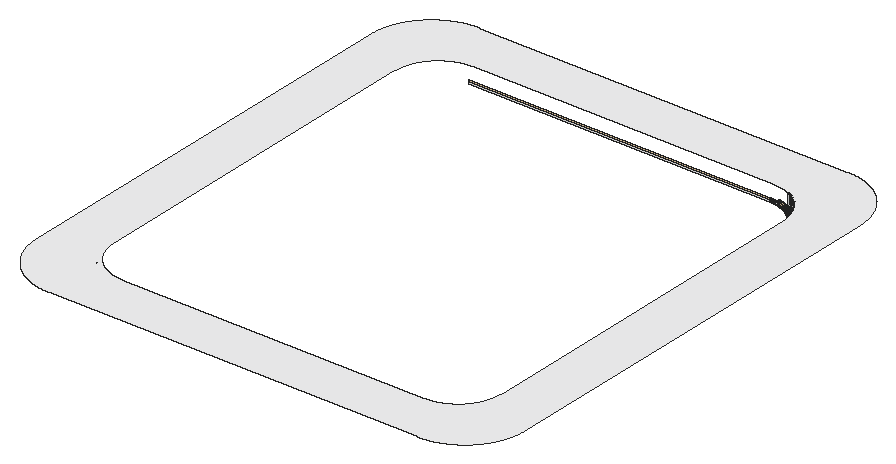
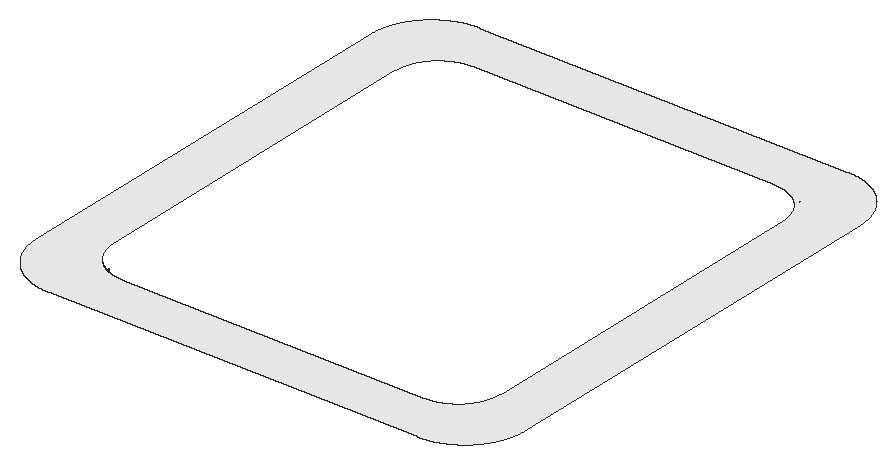
# SketchUp Ruby script. Lengths in inches.
U = 1.inch
M = Sketchup.active_model
def pt(a) = Geom::Point3d.new(a.map { |v| v * U })
def face(e, loops, mat)
  f = e.add_face(loops[0].map { |a| pt(a) })
  loops[1..].each { |l| e.add_face(l.map { |a| pt(a) }).erase! }
  f.material = f.back_material = mat if mat
  f
end
# faces: each face lists its corners as indices into pts; further lists are holes
def faces(e, pts, list, mat = nil) = list.each { |f| face(e, (f[0].is_a?(Array) ? f : [f]).map { |l| l.map { |i| pts[i] } }, mat) }
# xy, xz, yz: faces in a plane at the given z, y or x. An outline is a flat list of corners, or four numbers for a rectangle; further outlines are holes
def ring(l) = l.size == 4 ? [[l[0], l[1]], [l[2], l[1]], [l[2], l[3]], [l[0], l[3]]] : l.each_slice(2).to_a
def flat(e, list, mat, &to3) = list.each { |f| face(e, (f[0].is_a?(Array) ? f : [f]).map { |l| ring(l).map { |u, v| to3.(u, v) } }, mat) }
def xy(e, z, list, mat = nil) = flat(e, list, mat) { |x, y| [x, y, z] }
def xz(e, y, list, mat = nil) = flat(e, list, mat) { |x, z| [x, y, z] }
def yz(e, x, list, mat = nil) = flat(e, list, mat) { |y, z| [x, y, z] }
def lines(e, pts, list) = list.each { |a, b| e.add_line(pt(pts[a]), pt(pts[b])) }
# prism: a flat outline (further loops are holes) pulled along v
def prism(e, loops, v, mat = nil)
  f = face(e, loops, mat); d = Geom::Vector3d.new(v.map { |x| x * U })
  f.pushpull(f.normal.samedirection?(d) ? d.length : -d.length)
end
def box(e, o, s, mat = nil) = prism(e, [[o, [o[0] + s[0], o[1], o[2]], [o[0] + s[0], o[1] + s[1], o[2]], [o[0], o[1] + s[1], o[2]]]], [0, 0, s[2]], mat)
def at(x, y, z, deg = 0) = Geom::Transformation.translation(pt([x, y, z])) * Geom::Transformation.rotation(ORIGIN, Z_AXIS, deg.degrees)
def axes(o, x, y, z) = Geom::Transformation.new([*x, 0, *y, 0, *z, 0, *pt(o).to_a, 1])
def part(name) = M.definitions.add(name)
# library, detail: a bought-in or finely detailed component or shape, given as its bounding box
def library(name, o, s) = part(name).tap { |d| box(d.entities, o, s) }
def detail(e, o, s) = box(e.add_group.entities, o, s)
def put(e, d, t, mat = nil) = e.add_instance(d, t).tap { |i| i.material = mat if mat }
def group(e, t, mat = nil) = e.add_group.tap { |g| g.transformation = t; g.material = mat if mat }.entities
root = M.entities
M.materials.add("False Ceiling Light").color = [254, 223, 179]
M.materials.add("[Quartz Light Grey]").color = [251, 251, 252]
xy(root,120,[[[45.007,44.5,176.993,44.5,177.225,44.501,177.45,44.505,177.675,44.511,177.9,44.519,178.125,44.529,178.35,44.542,178.575,44.558,178.799,44.575,179.023,44.595,179.247,44.618,179.471,44.643,179.695,44.67,179.918,44.699,180.141,44.731,180.363,44.765,180.586,44.801,180.807,44.84,181.029,44.881,181.25,44.924,181.47,44.97,181.69,45.018,181.91,45.068,182.128,45.121,182.347,45.175,182.565,45.233,182.782,45.292,182.998,45.354,183.214,45.418,183.429,45.484,183.644,45.552,183.858,45.623,184.071,45.696,184.283,45.771,184.494,45.848,184.705,45.928,184.915,46.01,185.124,46.094,185.332,46.18,185.539,46.268,185.745,46.359,185.95,46.451,186.154,46.546,186.357,46.643,186.56,46.742,186.761,46.843,186.961,46.947,187.16,47.052,187.358,47.159,187.554,47.269,187.75,47.38,187.944,47.494,188.138,47.61,188.33,47.727,188.52,47.847,188.71,47.969,188.898,48.092,189.085,48.218,189.27,48.345,189.455,48.475,189.637,48.606,189.819,48.739,189.999,48.875,190.177,49.012,190.355,49.151,190.53,49.291,190.705,49.434,190.877,49.578,191.049,49.725,191.218,49.873,191.386,50.022,191.553,50.174,191.718,50.327,191.881,50.482,192.043,50.639,192.203,50.797,192.361,50.957,192.518,51.119,192.673,51.282,192.826,51.447,192.978,51.614,193.127,51.782,193.275,51.951,193.422,52.123,193.566,52.295,193.709,52.47,193.849,52.645,193.988,52.823,194.125,53.001,194.261,53.181,194.394,53.363,194.525,53.545,194.655,53.73,194.782,53.915,194.908,54.102,195.031,54.29,195.153,54.48,195.273,54.67,195.39,54.862,195.506,55.056,195.62,55.25,195.731,55.446,195.841,55.642,195.948,55.84,196.053,56.039,196.157,56.239,196.258,56.44,196.357,56.643,196.454,56.846,196.549,57.05,196.641,57.255,196.732,57.461,196.82,57.668,196.906,57.876,196.99,58.085,197.072,58.295,197.152,58.506,197.229,58.717,197.304,58.929,197.377,59.142,197.448,59.356,197.516,59.571,197.582,59.786,197.646,60.002,197.708,60.218,197.767,60.435,197.825,60.653,197.879,60.872,197.932,61.09,197.982,61.31,198.03,61.53,198.076,61.75,198.119,61.971,198.16,62.193,198.199,62.414,198.235,62.637,198.269,62.859,198.301,63.082,198.33,63.305,198.357,63.529,198.382,63.753,198.405,63.977,198.425,64.201,198.442,64.425,198.458,64.65,198.471,64.875,198.481,65.1,198.489,65.325,198.495,65.55,198.499,65.775,198.5,66.007,198.5,215.993,198.499,216.225,198.495,216.45,198.489,216.675,198.481,216.9,198.471,217.125,198.458,217.35,198.442,217.575,198.425,217.799,198.405,218.023,198.382,218.247,198.357,218.471,198.33,218.695,198.301,218.918,198.269,219.141,198.235,219.363,198.199,219.586,198.16,219.807,198.119,220.029,198.076,220.25,198.03,220.47,197.982,220.69,197.932,220.91,197.879,221.128,197.825,221.347,197.767,221.565,197.708,221.782,197.646,221.998,197.582,222.214,197.516,222.429,197.448,222.644,197.377,222.858,197.304,223.071,197.229,223.283,197.152,223.494,197.072,223.705,196.99,223.915,196.906,224.124,196.82,224.332,196.732,224.539,196.641,224.745,196.549,224.95,196.454,225.154,196.357,225.357,196.258,225.56,196.157,225.761,196.053,225.961,195.948,226.16,195.841,226.358,195.731,226.554,195.62,226.75,195.506,226.944,195.39,227.138,195.273,227.33,195.153,227.52,195.031,227.71,194.908,227.898,194.782,228.085,194.655,228.27,194.525,228.455,194.394,228.637,194.261,228.819,194.125,228.999,193.988,229.177,193.849,229.355,193.709,229.53,193.566,229.705,193.422,229.877,193.275,230.049,193.127,230.218,192.978,230.386,192.826,230.553,192.673,230.718,192.518,230.881,192.361,231.043,192.203,231.203,192.043,231.361,191.881,231.518,191.718,231.673,191.553,231.826,191.386,231.978,191.218,232.127,191.049,232.275,190.877,232.422,190.705,232.566,190.53,232.709,190.355,232.849,190.177,232.988,189.999,233.125,189.819,233.261,189.637,233.394,189.455,233.525,189.27,233.655,189.085,233.782,188.898,233.908,188.71,234.031,188.52,234.153,188.33,234.273,188.138,234.39,187.944,234.506,187.75,234.62,187.554,234.731,187.358,234.841,187.16,234.948,186.961,235.053,186.761,235.157,186.56,235.258,186.357,235.357,186.154,235.454,185.95,235.549,185.745,235.641,185.539,235.732,185.332,235.82,185.124,235.906,184.915,235.99,184.705,236.072,184.494,236.152,184.283,236.229,184.071,236.304,183.858,236.377,183.644,236.448,183.429,236.516,183.214,236.582,182.998,236.646,182.782,236.708,182.565,236.767,182.347,236.825,182.128,236.879,181.91,236.932,181.69,236.982,181.47,237.03,181.25,237.076,181.029,237.119,180.807,237.16,180.586,237.199,180.363,237.235,180.141,237.269,179.918,237.301,179.695,237.33,179.471,237.357,179.247,237.382,179.023,237.405,178.799,237.425,178.575,237.442,178.35,237.458,178.125,237.471,177.9,237.481,177.675,237.489,177.45,237.495,177.225,237.499,176.993,237.5,45.007,237.5,44.775,237.499,44.55,237.495,44.325,237.489,44.1,237.481,43.875,237.471,43.65,237.458,43.425,237.442,43.201,237.425,42.977,237.405,42.753,237.382,42.529,237.357,42.305,237.33,42.082,237.301,41.859,237.269,41.637,237.235,41.414,237.199,41.193,237.16,40.971,237.119,40.75,237.076,40.53,237.03,40.31,236.982,40.09,236.932,39.872,236.879,39.653,236.825,39.435,236.767,39.218,236.708,39.002,236.646,38.786,236.582,38.571,236.516,38.356,236.448,38.142,236.377,37.929,236.304,37.717,236.229,37.506,236.152,37.295,236.072,37.085,235.99,36.876,235.906,36.668,235.82,36.461,235.732,36.255,235.641,36.05,235.549,35.846,235.454,35.643,235.357,35.44,235.258,35.239,235.157,35.039,235.053,34.84,234.948,34.642,234.841,34.446,234.731,34.25,234.62,34.056,234.506,33.862,234.39,33.67,234.273,33.48,234.153,33.29,234.031,33.102,233.908,32.915,233.782,32.73,233.655,32.545,233.525,32.363,233.394,32.181,233.261,32.001,233.125,31.823,232.988,31.645,232.849,31.47,232.709,31.295,232.566,31.123,232.422,30.951,232.275,30.782,232.127,30.614,231.978,30.447,231.826,30.282,231.673,30.119,231.518,29.957,231.361,29.797,231.203,29.639,231.043,29.482,230.881,29.327,230.718,29.174,230.553,29.022,230.386,28.873,230.218,28.725,230.049,28.578,229.877,28.434,229.705,28.291,229.53,28.151,229.355,28.012,229.177,27.875,228.999,27.739,228.819,27.606,228.637,27.475,228.455,27.345,228.27,27.218,228.085,27.092,227.898,26.969,227.71,26.847,227.52,26.727,227.33,26.61,227.138,26.494,226.944,26.38,226.75,26.269,226.554,26.159,226.358,26.052,226.16,25.947,225.961,25.843,225.761,25.742,225.56,25.643,225.357,25.546,225.154,25.451,224.95,25.359,224.745,25.268,224.539,25.18,224.332,25.094,224.124,25.01,223.915,24.928,223.705,24.848,223.494,24.771,223.283,24.696,223.071,24.623,222.858,24.552,222.644,24.484,222.429,24.418,222.214,24.354,221.998,24.292,221.782,24.233,221.565,24.175,221.347,24.121,221.128,24.068,220.91,24.018,220.69,23.97,220.47,23.924,220.25,23.881,220.029,23.84,219.807,23.801,219.586,23.765,219.363,23.731,219.141,23.699,218.918,23.67,218.695,23.643,218.471,23.618,218.247,23.595,218.023,23.575,217.799,23.558,217.575,23.542,217.35,23.529,217.125,23.519,216.9,23.511,216.675,23.505,216.45,23.501,216.225,23.5,215.993,23.5,66.007,23.501,65.775,23.505,65.55,23.511,65.325,23.519,65.1,23.529,64.875,23.542,64.65,23.558,64.425,23.575,64.201,23.595,63.977,23.618,63.753,23.643,63.529,23.67,63.305,23.699,63.082,23.731,62.859,23.765,62.637,23.801,62.414,23.84,62.193,23.881,61.971,23.924,61.75,23.97,61.53,24.018,61.31,24.068,61.09,24.121,60.872,24.175,60.653,24.233,60.435,24.292,60.218,24.354,60.002,24.418,59.786,24.484,59.571,24.552,59.356,24.623,59.142,24.696,58.929,24.771,58.717,24.848,58.506,24.928,58.295,25.01,58.085,25.094,57.876,25.18,57.668,25.268,57.461,25.359,57.255,25.451,57.05,25.546,56.846,25.643,56.643,25.742,56.44,25.843,56.239,25.947,56.039,26.052,55.84,26.159,55.642,26.269,55.446,26.38,55.25,26.494,55.056,26.61,54.862,26.727,54.67,26.847,54.48,26.969,54.29,27.092,54.102,27.218,53.915,27.345,53.73,27.475,53.545,27.606,53.363,27.739,53.181,27.875,53.001,28.012,52.823,28.151,52.645,28.291,52.47,28.434,52.295,28.578,52.123,28.725,51.951,28.873,51.782,29.022,51.614,29.174,51.447,29.327,51.282,29.482,51.119,29.639,50.957,29.797,50.797,29.957,50.639,30.119,50.482,30.282,50.327,30.447,50.174,30.614,50.022,30.782,49.873,30.951,49.725,31.123,49.578,31.295,49.434,31.47,49.291,31.645,49.151,31.823,49.012,32.001,48.875,32.181,48.739,32.363,48.606,32.545,48.475,32.73,48.345,32.915,48.218,33.102,48.092,33.29,47.969,33.48,47.847,33.67,47.727,33.862,47.61,34.056,47.494,34.25,47.38,34.446,47.269,34.642,47.159,34.84,47.052,35.039,46.947,35.239,46.843,35.44,46.742,35.643,46.643,35.846,46.546,36.05,46.451,36.255,46.359,36.461,46.268,36.668,46.18,36.876,46.094,37.085,46.01,37.295,45.928,37.506,45.848,37.717,45.771,37.929,45.696,38.142,45.623,38.356,45.552,38.571,45.484,38.786,45.418,39.002,45.354,39.218,45.292,39.435,45.233,39.653,45.175,39.872,45.121,40.09,45.068,40.31,45.018,40.53,44.97,40.75,44.924,40.971,44.881,41.193,44.84,41.414,44.801,41.637,44.765,41.859,44.731,42.082,44.699,42.305,44.67,42.529,44.643,42.753,44.618,42.977,44.595,43.201,44.575,43.425,44.558,43.65,44.542,43.875,44.529,44.1,44.519,44.325,44.511,44.55,44.505,44.775,44.501],[56.989,62.5,56.796,62.501,56.593,62.505,56.389,62.512,56.186,62.521,55.983,62.533,55.78,62.548,55.577,62.565,55.374,62.585,55.172,62.608,54.97,62.633,54.768,62.661,54.567,62.692,54.366,62.725,54.166,62.761,53.966,62.8,53.767,62.841,53.568,62.885,53.37,62.931,53.172,62.98,52.975,63.032,52.779,63.086,52.583,63.142,52.389,63.202,52.195,63.264,52.002,63.328,51.809,63.395,51.618,63.464,51.428,63.536,51.238,63.611,51.05,63.6875,50.862,63.767,50.676,63.849,50.49,63.933,50.306,64.02,50.123,64.109,49.941,64.2,49.761,64.294,49.581,64.391,49.403,64.489,49.227,64.59,49.051,64.693,48.877,64.799,48.704,64.907,48.533,65.017,48.363,65.129,48.195,65.244,48.028,65.36,47.863,65.479,47.699,65.6,47.537,65.724,47.377,65.849,47.218,65.976,47.061,66.106,46.906,66.237,46.752,66.371,46.6,66.507,46.45,66.644,46.302,66.784,46.156,66.925,46.011,67.068,45.868,67.214,45.728,67.361,45.589,67.51,45.452,67.661,45.317,67.813,45.185,67.967,45.054,68.123,44.925,68.281,44.799,68.441,44.674,68.602,44.552,68.764,44.432,68.929,44.314,69.095,44.198,69.262,44.084,69.431,43.973,69.601,43.863,69.773,43.756,69.946,43.652,70.121,43.549,70.297,43.449,70.474,43.352,70.653,43.257,70.833,43.164,71.014,43.073,71.196,42.985,71.38,42.899,71.564,42.816,71.75,42.735,71.937,42.657,72.125,42.581,72.313,42.507,72.503,42.436,72.694,42.368,72.886,42.302,73.078,42.239,73.272,42.178,73.466,42.119,73.661,42.064,73.857,42.011,74.054,41.96,74.251,41.912,74.449,41.867,74.647,41.824,74.846,41.784,75.046,41.746,75.246,41.712,75.446,41.679,75.647,41.65,75.849,41.623,76.051,41.599,76.253,41.577,76.455,41.558,76.658,41.542,76.861,41.528,77.064,41.517,77.267,41.509,77.47,41.503,77.674,41.5,77.878,41.5,204.011,41.501,204.203,41.505,204.406,41.512,204.609,41.521,204.811,41.533,205.014,41.548,205.216,41.565,205.418,41.585,205.62,41.607,205.822,41.633,206.023,41.66,206.224,41.691,206.425,41.724,206.625,41.759,206.825,41.798,207.024,41.839,207.223,41.882,207.421,41.928,207.618,41.977,207.815,42.028,208.012,42.082,208.207,42.138,208.402,42.197,208.596,42.259,208.79,42.323,208.982,42.389,209.174,42.458,209.365,42.529,209.555,42.603,209.744,42.68,209.932,42.759,210.119,42.84,210.304,42.924,210.489,43.01,210.673,43.098,210.856,43.189,211.037,43.283,211.217,43.378,211.396,43.476,211.574,43.577,211.75,43.679,211.925,43.784,212.099,43.891,212.271,44.001,212.442,44.112,212.611,44.226,212.779,44.342,212.946,44.46,213.111,44.581,213.274,44.703,213.436,44.828,213.596,44.954,213.755,45.083,213.911,45.214,214.066,45.346,214.22,45.481,214.372,45.618,214.521,45.757,214.67,45.897,214.816,46.04,214.96,46.184,215.103,46.33,215.243,46.479,215.382,46.628,215.519,46.78,215.654,46.934,215.786,47.089,215.917,47.245,216.046,47.404,216.172,47.564,216.297,47.726,216.419,47.889,216.54,48.054,216.658,48.221,216.774,48.389,216.888,48.558,216.999,48.729,217.109,48.901,217.216,49.075,217.321,49.25,217.423,49.426,217.524,49.604,217.622,49.783,217.717,49.963,217.811,50.144,217.902,50.327,217.99,50.511,218.076,50.696,218.16,50.881,218.241,51.068,218.32,51.256,218.397,51.445,218.471,51.635,218.542,51.826,218.611,52.018,218.677,52.21,218.741,52.404,218.803,52.598,218.862,52.793,218.918,52.988,218.972,53.185,219.023,53.382,219.072,53.579,219.118,53.777,219.161,53.976,219.202,54.175,219.241,54.375,219.276,54.575,219.309,54.776,219.34,54.977,219.367,55.178,219.393,55.38,219.415,55.582,219.435,55.784,219.452,55.986,219.467,56.189,219.479,56.391,219.488,56.594,219.495,56.797,219.499,56.989,219.5,165.011,219.5,165.203,219.499,165.406,219.495,165.609,219.488,165.811,219.479,166.014,219.467,166.216,219.452,166.418,219.435,166.62,219.415,166.822,219.393,167.023,219.367,167.224,219.34,167.425,219.309,167.625,219.276,167.825,219.241,168.024,219.202,168.223,219.161,168.421,219.118,168.618,219.072,168.815,219.023,169.012,218.972,169.207,218.918,169.402,218.862,169.596,218.803,169.79,218.741,169.982,218.677,170.174,218.611,170.365,218.542,170.555,218.471,170.744,218.397,170.932,218.32,171.119,218.241,171.304,218.16,171.489,218.076,171.673,217.99,171.856,217.902,172.037,217.811,172.217,217.717,172.396,217.622,172.574,217.524,172.75,217.423,172.925,217.321,173.099,217.216,173.271,217.109,173.442,216.999,173.611,216.888,173.779,216.774,173.946,216.658,174.111,216.54,174.274,216.419,174.436,216.297,174.596,216.172,174.755,216.046,174.911,215.917,175.066,215.786,175.22,215.654,175.372,215.519,175.521,215.382,175.67,215.243,175.816,215.103,175.96,214.96,176.103,214.816,176.243,214.67,176.382,214.521,176.519,214.372,176.654,214.22,176.786,214.066,176.917,213.911,177.046,213.755,177.172,213.596,177.297,213.436,177.419,213.274,177.54,213.111,177.658,212.946,177.774,212.779,177.888,212.611,177.999,212.442,178.109,212.271,178.216,212.099,178.321,211.925,178.423,211.75,178.524,211.574,178.622,211.396,178.717,211.217,178.811,211.037,178.902,210.856,178.99,210.673,179.076,210.489,179.16,210.304,179.241,210.119,179.32,209.932,179.397,209.744,179.471,209.555,179.542,209.365,179.611,209.174,179.677,208.982,179.741,208.79,179.803,208.596,179.862,208.402,179.918,208.207,179.972,208.012,180.023,207.815,180.072,207.618,180.118,207.421,180.161,207.223,180.202,207.024,180.241,206.825,180.276,206.625,180.309,206.425,180.34,206.224,180.367,206.023,180.393,205.822,180.415,205.62,180.435,205.418,180.452,205.216,180.467,205.014,180.479,204.811,180.488,204.609,180.495,204.406,180.499,204.203,180.5,204.011,180.5,77.989,180.499,77.797,180.495,77.594,180.488,77.391,180.479,77.189,180.467,76.986,180.452,76.784,180.435,76.582,180.415,76.38,180.393,76.178,180.367,75.977,180.34,75.776,180.309,75.575,180.276,75.375,180.241,75.175,180.202,74.976,180.161,74.777,180.118,74.579,180.072,74.382,180.023,74.185,179.972,73.988,179.918,73.793,179.862,73.598,179.803,73.404,179.741,73.21,179.677,73.018,179.611,72.826,179.542,72.635,179.471,72.445,179.397,72.256,179.32,72.068,179.241,71.881,179.16,71.696,179.076,71.511,178.99,71.327,178.902,71.144,178.811,70.963,178.717,70.783,178.622,70.604,178.524,70.426,178.423,70.25,178.321,70.075,178.216,69.901,178.109,69.729,177.999,69.558,177.888,69.389,177.774,69.221,177.658,69.054,177.54,68.889,177.419,68.726,177.297,68.564,177.172,68.404,177.046,68.245,176.917,68.089,176.786,67.934,176.654,67.78,176.519,67.628,176.382,67.479,176.243,67.33,176.103,67.184,175.96,67.04,175.816,66.897,175.67,66.757,175.521,66.618,175.372,66.481,175.22,66.346,175.066,66.214,174.911,66.083,174.755,65.954,174.596,65.828,174.436,65.703,174.274,65.581,174.111,65.46,173.946,65.342,173.779,65.226,173.611,65.112,173.442,65.001,173.271,64.891,173.099,64.784,172.925,64.679,172.75,64.577,172.574,64.476,172.396,64.378,172.217,64.283,172.037,64.189,171.856,64.098,171.673,64.01,171.489,63.924,171.304,63.84,171.119,63.759,170.932,63.68,170.744,63.603,170.555,63.529,170.365,63.458,170.174,63.389,169.982,63.323,169.79,63.259,169.596,63.197,169.402,63.138,169.207,63.082,169.012,63.028,168.815,62.977,168.618,62.928,168.421,62.882,168.223,62.839,168.024,62.798,167.825,62.759,167.625,62.724,167.425,62.691,167.224,62.66,167.023,62.633,166.822,62.607,166.62,62.585,166.418,62.565,166.216,62.548,166.014,62.533,165.811,62.521,165.609,62.512,165.406,62.505,165.203,62.501,165.011,62.5],[45,66,45,66.063,45.004,66]]],"[Quartz Light Grey]")
xz(root,217.5,[[56.995,115.32,165.005,116.49]],"False Ceiling Light")
xz(root,217.5,[[56.995,115.32,165.005,115.905]],"[Quartz Light Grey]")
p = [[176.025,211.791,115.32],[176.126,211.647,115.32],[176.126,211.647,116.49],[176.025,211.791,116.49],[176.126,211.647,115.32],[176.025,211.791,115.32],
  [176.025,211.791,115.905],[176.126,211.647,115.905],[175.922,211.935,115.32],[175.922,211.935,116.49],[175.922,211.935,115.32],[175.922,211.935,115.905],
  [175.817,212.077,115.32],[175.817,212.077,116.49],[175.817,212.077,115.32],[175.817,212.077,115.905],[175.71,212.218,115.32],[175.71,212.218,116.49],
  [175.71,212.218,115.32],[175.71,212.218,115.905],[175.602,212.358,115.32],[175.602,212.358,116.49],[175.602,212.358,115.32],[175.602,212.358,115.905],
  [175.491,212.496,115.32],[175.491,212.496,116.49],[175.491,212.496,115.32],[175.491,212.496,115.905],[175.379,212.632,115.32],[175.379,212.632,116.49],
  [175.379,212.632,115.32],[175.379,212.632,115.905],[175.266,212.768,115.32],[175.266,212.768,116.49],[175.266,212.768,115.32],[175.266,212.768,115.905],
  [175.15,212.901,115.32],[175.15,212.901,116.49],[175.15,212.901,115.32],[175.15,212.901,115.905],[175.032,213.033,115.32],[175.032,213.033,116.49],
  [175.032,213.033,115.32],[175.032,213.033,115.905],[174.913,213.164,115.32],[174.913,213.164,116.49],[174.913,213.164,115.32],[174.913,213.164,115.905],
  [174.793,213.293,115.32],[174.793,213.293,116.49],[174.793,213.293,115.32],[174.793,213.293,115.905],[174.67,213.42,115.32],[174.67,213.42,116.49],
  [174.67,213.42,115.32],[174.67,213.42,115.905],[176.148,213.272,115.32],[176.026,213.417,115.32],[176.026,213.417,116.49],[176.148,213.272,116.49],
  [174.546,213.546,115.32],[174.546,213.546,116.49],[174.546,213.546,115.32],[174.546,213.546,115.905],[175.902,213.561,115.32],[175.902,213.561,116.49],
  [174.42,213.67,115.32],[174.42,213.67,116.49],[174.42,213.67,115.32],[174.42,213.67,115.905],[175.776,213.702,115.32],[175.776,213.702,116.49],
  [174.293,213.793,115.32],[174.293,213.793,116.49],[174.293,213.793,115.32],[174.293,213.793,115.905],[175.648,213.843,115.32],[175.648,213.843,116.49],
  [174.164,213.913,115.32],[174.164,213.913,116.49],[174.164,213.913,115.32],[174.164,213.913,115.905],[175.518,213.981,115.32],[175.518,213.981,116.49],
  [174.033,214.032,115.32],[174.033,214.032,116.49],[174.033,214.032,115.32],[174.033,214.032,115.905],[173.901,214.15,115.32],[173.901,214.15,116.49],
  [173.901,214.15,115.32],[173.901,214.15,115.905],[175.386,214.118,115.32],[175.386,214.118,116.49],[173.768,214.266,115.32],[173.768,214.266,116.49],
  [173.768,214.266,115.32],[173.768,214.266,115.905],[175.253,214.253,115.32],[175.253,214.253,116.49],[173.632,214.379,115.32],[173.632,214.379,116.49],
  [173.632,214.379,115.32],[173.632,214.379,115.905],[175.118,214.386,115.32],[175.118,214.386,116.49],[173.496,214.491,115.32],[173.496,214.491,116.49],
  [173.496,214.491,115.32],[173.496,214.491,115.905],[174.981,214.518,115.32],[174.981,214.518,116.49],[173.358,214.602,115.32],[173.358,214.602,116.49],
  [173.358,214.602,115.32],[173.358,214.602,115.905],[174.843,214.648,115.32],[174.843,214.648,116.49],[173.218,214.71,115.32],[173.218,214.71,116.49],
  [173.218,214.71,115.32],[173.218,214.71,115.905],[174.702,214.776,115.32],[174.702,214.776,116.49],[173.077,214.817,115.32],[173.077,214.817,116.49],
  [173.077,214.817,115.32],[173.077,214.817,115.905],[176.103,214.816,115.32],[176.243,214.67,115.32],[176.243,214.67,120],[176.103,214.816,120],
  [172.935,214.922,115.32],[172.935,214.922,116.49],[172.935,214.922,115.32],[172.935,214.922,115.905],[174.561,214.902,115.32],[174.561,214.902,116.49],
  [175.96,214.96,115.32],[175.96,214.96,120],[172.791,215.025,115.32],[172.791,215.025,116.49],[172.791,215.025,115.32],[172.791,215.025,115.905],
  [174.417,215.026,115.32],[174.417,215.026,116.49],[172.647,215.126,115.32],[172.647,215.126,116.49],[172.647,215.126,115.32],[172.647,215.126,115.905],
  [174.272,215.148,115.32],[174.272,215.148,116.49],[175.816,215.103,115.32],[175.816,215.103,120],[172.5,215.225,115.32],[172.5,215.225,116.49],
  [172.5,215.225,115.32],[172.5,215.225,115.905],[174.125,215.269,115.32],[174.125,215.269,116.49],[175.67,215.243,115.32],[175.67,215.243,120],
  [172.353,215.322,115.32],[172.353,215.322,116.49],[172.353,215.322,115.32],[172.353,215.322,115.905],[175.521,215.382,115.32],[175.521,215.382,120],
  [172.204,215.417,115.32],[172.204,215.417,116.49],[172.204,215.417,115.32],[172.204,215.417,115.905],[173.977,215.387,115.32],[173.977,215.387,116.49],
  [172.054,215.511,115.32],[172.054,215.511,116.49],[172.054,215.511,115.32],[172.054,215.511,115.905],[173.827,215.504,115.32],[173.827,215.504,116.49],
  [175.372,215.519,115.32],[175.372,215.519,120],[171.902,215.602,115.32],[171.902,215.602,116.49],[171.902,215.602,115.32],[171.902,215.602,115.905],
  [173.676,215.618,115.32],[173.676,215.618,116.49],[175.22,215.654,115.32],[175.22,215.654,120],[171.75,215.691,115.32],[171.75,215.691,116.49],
  [171.75,215.691,115.32],[171.75,215.691,115.905],[173.523,215.731,115.32],[173.523,215.731,116.49],[171.596,215.779,115.32],[171.596,215.779,116.49],
  [171.596,215.779,115.32],[171.596,215.779,115.905],[173.369,215.841,115.32],[173.369,215.841,116.49],[175.066,215.786,115.32],[175.066,215.786,120],
  [171.442,215.864,115.32],[171.442,215.864,116.49],[171.442,215.864,115.32],[171.442,215.864,115.905],[173.213,215.95,115.32],[173.213,215.95,116.49],
  [174.911,215.917,115.32],[174.911,215.917,120],[171.129,216.029,115.32],[171.286,215.947,115.32],[171.286,215.947,116.49],[171.129,216.029,116.49],
  [171.286,215.947,115.32],[171.129,216.029,115.32],[171.129,216.029,115.905],[171.286,215.947,115.905],[173.056,216.056,115.32],[173.056,216.056,116.49],
  [174.755,216.046,115.32],[174.755,216.046,120],[170.971,216.108,115.32],[170.971,216.108,116.49],[170.971,216.108,115.32],[170.971,216.108,115.905],
  [174.596,216.172,115.32],[174.596,216.172,120],[170.812,216.185,115.32],[170.812,216.185,116.49],[170.812,216.185,115.32],[170.812,216.185,115.905],
  [172.897,216.161,115.32],[172.897,216.161,116.49],[170.652,216.26,115.32],[170.652,216.26,116.49],[170.652,216.26,115.32],[170.652,216.26,115.905],
  [172.737,216.263,115.32],[172.737,216.263,116.49],[174.436,216.297,115.32],[174.436,216.297,120],[170.329,216.404,115.32],[170.491,216.333,115.32],
  [170.491,216.333,116.49],[170.329,216.404,116.49],[170.491,216.333,115.32],[170.329,216.404,115.32],[170.329,216.404,115.905],[170.491,216.333,115.905],
  [172.576,216.363,115.32],[172.576,216.363,116.49],[174.274,216.419,115.32],[174.274,216.419,120],[170.166,216.472,115.32],[170.166,216.472,116.49],
  [170.166,216.472,115.32],[170.166,216.472,115.905],[172.414,216.461,115.32],[172.414,216.461,116.49],[174.111,216.54,115.32],[174.111,216.54,120],
  [169.838,216.603,115.32],[170.003,216.539,115.32],[170.003,216.539,116.49],[169.838,216.603,116.49],[170.003,216.539,115.32],[169.838,216.603,115.32],
  [169.838,216.603,115.905],[170.003,216.539,115.905],[172.25,216.557,115.32],[172.25,216.557,116.49],[173.946,216.658,115.32],[173.946,216.658,120],
  [169.673,216.666,115.32],[169.673,216.666,116.49],[169.673,216.666,115.32],[169.673,216.666,115.905],[172.085,216.651,115.32],[172.085,216.651,116.49],
  [169.339,216.784,115.32],[169.506,216.726,115.32],[169.506,216.726,116.49],[169.339,216.784,116.49],[169.506,216.726,115.32],[169.339,216.784,115.32],
  [169.339,216.784,115.905],[169.506,216.726,115.905],[171.919,216.743,115.32],[171.751,216.832,115.32],[171.751,216.832,116.49],[171.919,216.743,116.49],
  [173.779,216.774,115.32],[173.779,216.774,120],[169.003,216.893,115.32],[169.172,216.839,115.32],[169.172,216.839,116.49],[169.003,216.893,116.49],
  [169.172,216.839,115.32],[169.003,216.893,115.32],[169.003,216.893,115.905],[169.172,216.839,115.905],[171.583,216.92,115.32],[171.583,216.92,116.49],
  [173.611,216.888,115.32],[173.611,216.888,120],[168.664,216.993,115.32],[168.834,216.944,115.32],[168.834,216.944,116.49],[168.664,216.993,116.49],
  [168.834,216.944,115.32],[168.664,216.993,115.32],[168.664,216.993,115.905],[168.834,216.944,115.905],[171.413,217.005,115.32],[171.413,217.005,116.49],
  [173.442,216.999,115.32],[173.442,216.999,120],[168.323,217.085,115.32],[168.494,217.04,115.32],[168.494,217.04,116.49],[168.323,217.085,116.49],
  [168.494,217.04,115.32],[168.323,217.085,115.32],[168.323,217.085,115.905],[168.494,217.04,115.905],[171.242,217.088,115.32],[171.242,217.088,116.49],
  [173.271,217.109,115.32],[173.271,217.109,120],[167.979,217.167,115.32],[168.152,217.127,115.32],[168.152,217.127,116.49],[167.979,217.167,116.49],
  [168.152,217.127,115.32],[167.979,217.167,115.32],[167.979,217.167,115.905],[168.152,217.127,115.905],[171.071,217.168,115.32],[171.071,217.168,116.49],
  [173.099,217.216,115.32],[173.099,217.216,120],[167.46,217.274,115.32],[167.634,217.241,115.32],[167.634,217.241,116.49],[167.46,217.274,116.49],
  [167.634,217.241,115.32],[167.46,217.274,115.32],[167.46,217.274,115.905],[167.634,217.241,115.905],[167.807,217.205,115.32],[167.807,217.205,116.49],
  [167.807,217.205,115.32],[167.807,217.205,115.905],[170.898,217.246,115.32],[170.724,217.323,115.32],[170.724,217.323,116.49],[170.898,217.246,116.49],
  [172.925,217.321,115.32],[172.925,217.321,120],[166.937,217.36,115.32],[167.112,217.334,115.32],[167.112,217.334,116.49],[166.937,217.36,116.49],
  [167.112,217.334,115.32],[166.937,217.36,115.32],[166.937,217.36,115.905],[167.112,217.334,115.905],[167.286,217.305,115.32],[167.286,217.305,116.49],
  [167.286,217.305,115.32],[167.286,217.305,115.905],[170.549,217.396,115.32],[170.549,217.396,116.49],[172.75,217.423,115.32],[172.75,217.423,120],
  [166.059,217.458,115.32],[166.235,217.443,115.32],[166.235,217.443,116.49],[166.059,217.458,116.49],[166.235,217.443,115.32],[166.059,217.458,115.32],
  [166.059,217.458,115.905],[166.235,217.443,115.905],[166.411,217.426,115.32],[166.411,217.426,116.49],[166.411,217.426,115.32],[166.411,217.426,115.905],
  [166.587,217.406,115.32],[166.587,217.406,116.49],[166.587,217.406,115.32],[166.587,217.406,115.905],[166.762,217.385,115.32],[166.762,217.385,116.49],
  [166.762,217.385,115.32],[166.762,217.385,115.905],[170.373,217.468,115.32],[170.373,217.468,116.49],[172.574,217.524,115.32],[172.574,217.524,120],
  [165.005,217.5,115.32],[165.177,217.499,115.32],[165.177,217.499,116.49],[165.005,217.5,116.49],[165.177,217.499,115.32],[165.005,217.5,115.32],
  [165.005,217.5,115.905],[165.177,217.499,115.905],[165.353,217.495,115.32],[165.353,217.495,116.49],[165.353,217.495,115.32],[165.353,217.495,115.905],
  [165.53,217.49,115.32],[165.53,217.49,116.49],[165.53,217.49,115.32],[165.53,217.49,115.905],[165.707,217.482,115.32],[165.707,217.482,116.49],
  [165.707,217.482,115.32],[165.707,217.482,115.905],[165.883,217.471,115.32],[165.883,217.471,116.49],[165.883,217.471,115.32],[165.883,217.471,115.905],
  [170.196,217.537,115.32],[170.019,217.604,115.32],[170.019,217.604,116.49],[170.196,217.537,116.49],[172.396,217.622,115.32],[172.396,217.622,120],
  [169.84,217.668,115.32],[169.84,217.668,116.49],[172.217,217.717,115.32],[172.217,217.717,120],[169.661,217.731,115.32],[169.481,217.79,115.32],
  [169.481,217.79,116.49],[169.661,217.731,116.49],[172.037,217.811,115.32],[172.037,217.811,120],[169.3,217.848,115.32],[169.118,217.903,115.32],
  [169.118,217.903,116.49],[169.3,217.848,116.49],[171.856,217.902,115.32],[171.856,217.902,120],[168.936,217.956,115.32],[168.936,217.956,116.49],
  [171.673,217.99,115.32],[171.673,217.99,120],[168.753,218.006,115.32],[168.569,218.054,115.32],[168.569,218.054,116.49],[168.753,218.006,116.49],
  [171.489,218.076,115.32],[171.489,218.076,120],[168.2,218.143,115.32],[168.015,218.183,115.32],[168.015,218.183,116.49],[168.2,218.143,116.49],
  [168.385,218.099,115.32],[168.385,218.099,116.49],[171.304,218.16,115.32],[171.304,218.16,120],[167.829,218.221,115.32],[167.642,218.257,115.32],
  [167.642,218.257,116.49],[167.829,218.221,116.49],[171.119,218.241,115.32],[171.119,218.241,120]]
faces(root,p,[[0,1,2,3],[8,0,3,9],[12,8,9,13],[16,12,13,17],[20,16,17,21],[24,20,21,25],[28,24,25,29],[32,28,29,33],
  [36,32,33,37],[40,36,37,41],[44,40,41,45],[48,44,45,49],[52,48,49,53],[56,57,58,59],[60,52,53,61],[57,64,65,58],
  [66,60,61,67],[64,70,71,65],[72,66,67,73],[70,76,77,71],[78,72,73,79],[76,82,83,77],[84,78,79,85],[88,84,85,89],
  [82,92,93,83],[94,88,89,95],[92,98,99,93],[100,94,95,101],[98,104,105,99],[106,100,101,107],[104,110,111,105],[112,106,107,113],
  [110,116,117,111],[118,112,113,119],[116,122,123,117],[124,118,119,125],[132,124,125,133],[122,136,137,123],[140,132,133,141],[136,144,145,137],
  [146,140,141,147],[144,150,151,145],[154,146,147,155],[150,158,159,151],[162,154,155,163],[168,162,163,169],[158,172,173,159],[174,168,169,175],
  [172,178,179,173],[182,174,175,183],[178,186,187,179],[190,182,183,191],[186,194,195,187],[196,190,191,197],[194,200,201,195],[204,196,197,205],
  [200,208,209,201],[212,213,214,215],[213,204,205,214],[208,220,221,209],[224,212,215,225],[230,224,225,231],[220,234,235,221],[236,230,231,237],
  [234,240,241,235],[244,245,246,247],[245,236,237,246],[240,252,253,241],[256,244,247,257],[252,260,261,253],[264,265,266,267],[265,256,257,266],
  [260,272,273,261],[276,264,267,277],[272,280,281,273],[282,283,284,285],[283,276,277,284],[290,291,292,293],[280,290,293,281],[296,297,298,299],
  [297,282,285,298],[291,304,305,292],[308,309,310,311],[309,296,299,310],[304,316,317,305],[320,321,322,323],[321,308,311,322],[316,328,329,317],
  [332,333,334,335],[333,320,323,334],[328,340,341,329],[344,345,346,347],[345,352,353,346],[352,332,335,353],[356,357,358,359],[340,356,359,341],
  [362,363,364,365],[363,370,371,364],[370,344,347,371],[357,374,375,358],[378,379,380,381],[379,386,387,380],[386,390,391,387],[390,394,395,391],
  [394,362,365,395],[374,398,399,375],[402,403,404,405],[403,410,411,404],[410,414,415,411],[414,418,419,415],[418,422,423,419],[422,378,381,423],
  [426,427,428,429],[398,426,429,399],[427,432,433,428],[436,437,438,439],[432,436,439,433],[442,443,444,445],[437,442,445,438],[443,448,449,444],
  [452,453,454,455],[448,452,455,449],[458,459,460,461],[462,458,461,463],[453,462,463,454],[466,467,468,469],[459,466,469,460]],"False Ceiling Light")
faces(root,p,[[4,5,6,7],[5,10,11,6],[10,14,15,11],[14,18,19,15],[18,22,23,19],[22,26,27,23],[26,30,31,27],[30,34,35,31],
  [34,38,39,35],[38,42,43,39],[42,46,47,43],[46,50,51,47],[50,54,55,51],[54,62,63,55],[62,68,69,63],[68,74,75,69],
  [74,80,81,75],[80,86,87,81],[86,90,91,87],[90,96,97,91],[96,102,103,97],[102,108,109,103],[108,114,115,109],[114,120,121,115],
  [120,126,127,121],[128,129,130,131],[126,134,135,127],[138,128,131,139],[134,142,143,135],[142,148,149,143],[152,138,139,153],[148,156,157,149],
  [160,152,153,161],[156,164,165,157],[166,160,161,167],[164,170,171,165],[170,176,177,171],[180,166,167,181],[176,184,185,177],[188,180,181,189],
  [184,192,193,185],[192,198,199,193],[202,188,189,203],[198,206,207,199],[210,202,203,211],[216,217,218,219],[206,216,219,207],[222,210,211,223],
  [217,226,227,218],[228,222,223,229],[226,232,233,227],[232,238,239,233],[242,228,229,243],[248,249,250,251],[238,248,251,239],[254,242,243,255],
  [249,258,259,250],[262,254,255,263],[268,269,270,271],[258,268,271,259],[274,262,263,275],[269,278,279,270],[286,287,288,289],[278,286,289,279],
  [294,274,275,295],[300,301,302,303],[287,300,303,288],[306,294,295,307],[312,313,314,315],[301,312,315,302],[318,306,307,319],[324,325,326,327],
  [313,324,327,314],[330,318,319,331],[336,337,338,339],[325,336,339,326],[342,330,331,343],[348,349,350,351],[354,348,351,355],[337,354,355,338],
  [360,342,343,361],[366,367,368,369],[372,366,369,373],[349,372,373,350],[376,360,361,377],[382,383,384,385],[388,382,385,389],[392,388,389,393],
  [396,392,393,397],[367,396,397,368],[400,376,377,401],[406,407,408,409],[412,406,409,413],[416,412,413,417],[420,416,417,421],[424,420,421,425],
  [383,424,425,384],[430,400,401,431],[434,430,431,435],[440,434,435,441],[446,440,441,447],[450,446,447,451],[456,450,451,457],[464,456,457,465],
  [470,464,465,471]],"[Quartz Light Grey]")
